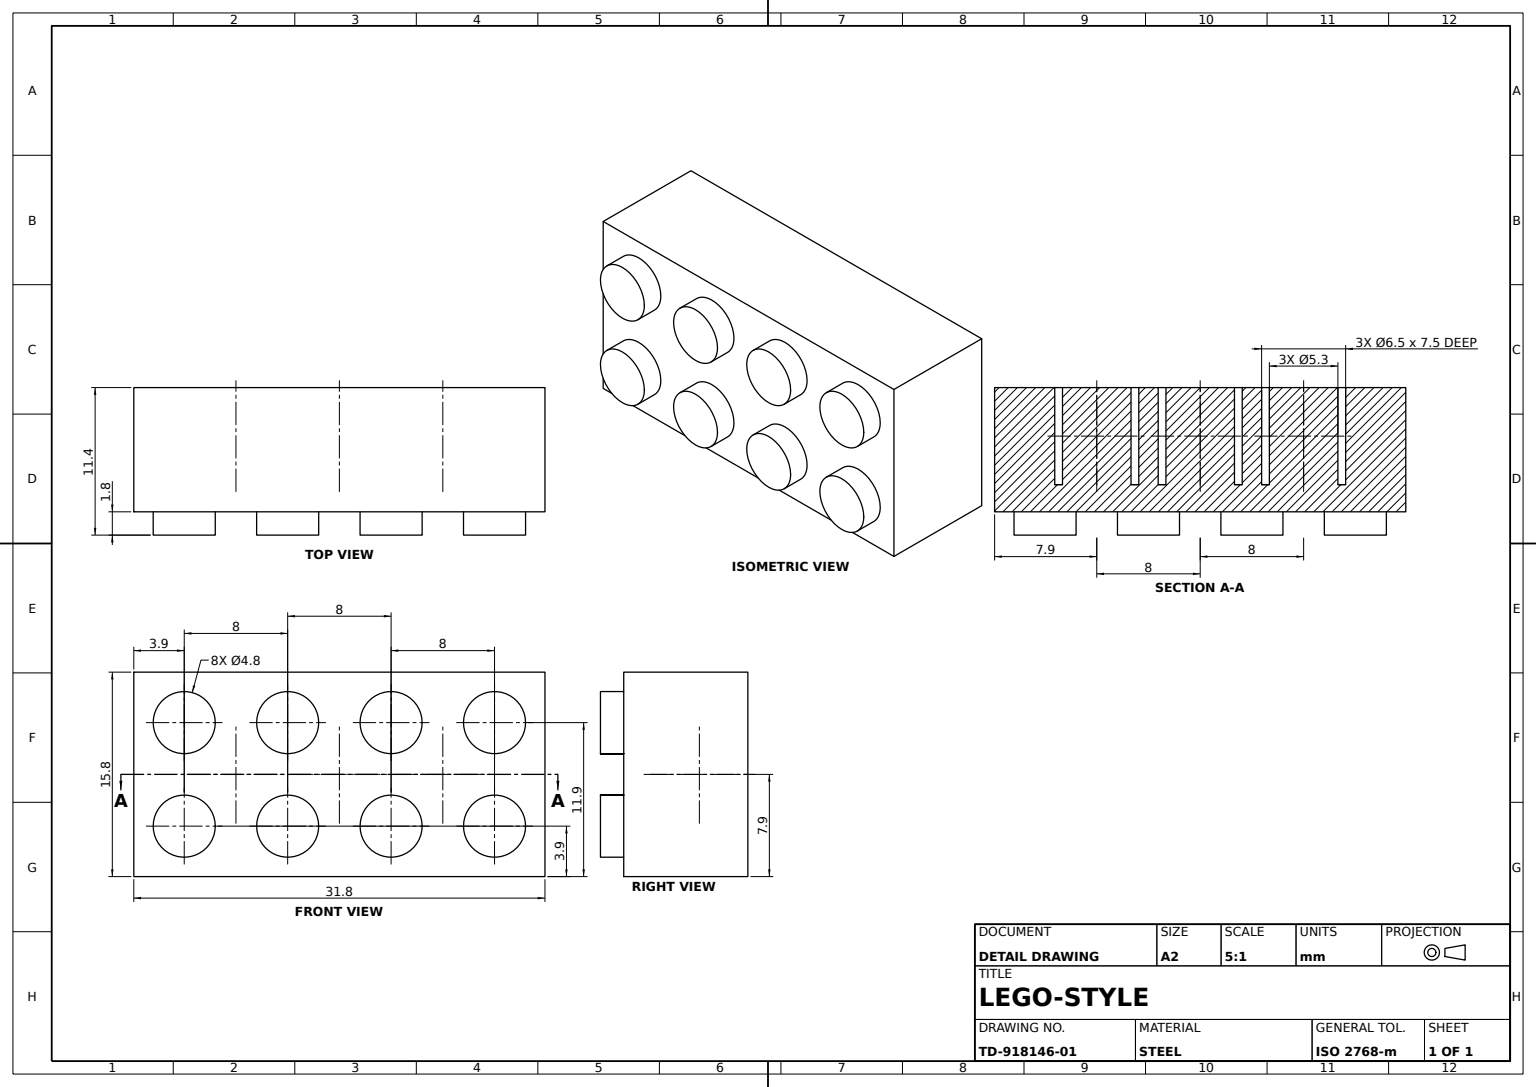
ISO-10303-21;
HEADER;
FILE_DESCRIPTION((''),'2;1');
FILE_NAME('','',(''),(''),'','','');
FILE_SCHEMA(('AUTOMOTIVE_DESIGN'));
ENDSEC;
DATA;
#1=APPLICATION_CONTEXT('');
#2=PRODUCT_CONTEXT('',#1,'mechanical');
#3=PRODUCT('','','',(#2));
#4=PRODUCT_DEFINITION_FORMATION('','',#3);
#5=PRODUCT_DEFINITION_CONTEXT('',#1,'design');
#6=PRODUCT_DEFINITION('','',#4,#5);
#7=PRODUCT_DEFINITION_SHAPE('','',#6);
#8=(LENGTH_UNIT()NAMED_UNIT(*)SI_UNIT(.MILLI.,.METRE.));
#9=(NAMED_UNIT(*)PLANE_ANGLE_UNIT()SI_UNIT($,.RADIAN.));
#10=(NAMED_UNIT(*)SI_UNIT($,.STERADIAN.)SOLID_ANGLE_UNIT());
#11=UNCERTAINTY_MEASURE_WITH_UNIT(LENGTH_MEASURE(1.E-05),#8,'distance_accuracy_value','');
#12=(GEOMETRIC_REPRESENTATION_CONTEXT(3)GLOBAL_UNCERTAINTY_ASSIGNED_CONTEXT((#11))GLOBAL_UNIT_ASSIGNED_CONTEXT((#8,#9,#10))REPRESENTATION_CONTEXT('',''));
#13=CARTESIAN_POINT('',(-4.75,0.,7.5));
#14=VERTEX_POINT('',#13);
#15=CARTESIAN_POINT('',(-11.25,0.,7.5));
#16=VERTEX_POINT('',#15);
#17=CARTESIAN_POINT('',(-8.,0.,7.5));
#18=DIRECTION('',(0.,0.,-1.));
#19=DIRECTION('',(-1.,0.,0.));
#20=AXIS2_PLACEMENT_3D('',#17,#18,#19);
#21=CIRCLE('',#20,3.25);
#22=EDGE_CURVE('',#14,#16,#21,.T.);
#23=ORIENTED_EDGE('',*,*,#22,.T.);
#24=EDGE_CURVE('',#16,#14,#21,.T.);
#25=ORIENTED_EDGE('',*,*,#24,.T.);
#26=EDGE_LOOP('',(#23,#25));
#27=FACE_OUTER_BOUND('',#26,.T.);
#28=CARTESIAN_POINT('',(-5.35,0.,7.5));
#29=VERTEX_POINT('',#28);
#30=CARTESIAN_POINT('',(-10.65,0.,7.5));
#31=VERTEX_POINT('',#30);
#32=CIRCLE('',#20,2.65);
#33=EDGE_CURVE('',#29,#31,#32,.T.);
#34=ORIENTED_EDGE('',*,*,#33,.F.);
#35=EDGE_CURVE('',#31,#29,#32,.T.);
#36=ORIENTED_EDGE('',*,*,#35,.F.);
#37=EDGE_LOOP('',(#34,#36));
#38=FACE_BOUND('',#37,.T.);
#39=PLANE('',#20);
#40=ADVANCED_FACE('',(#27,#38),#39,.T.);
#41=CARTESIAN_POINT('',(-6.4,4.,11.4));
#42=VERTEX_POINT('',#41);
#43=CARTESIAN_POINT('',(-1.6,4.,11.4));
#44=VERTEX_POINT('',#43);
#45=CARTESIAN_POINT('',(-4.,4.,11.4));
#46=DIRECTION('',(0.,0.,1.));
#47=DIRECTION('',(1.,0.,0.));
#48=AXIS2_PLACEMENT_3D('',#45,#46,#47);
#49=CIRCLE('',#48,2.4);
#50=EDGE_CURVE('',#42,#44,#49,.T.);
#51=ORIENTED_EDGE('',*,*,#50,.T.);
#52=EDGE_CURVE('',#44,#42,#49,.T.);
#53=ORIENTED_EDGE('',*,*,#52,.T.);
#54=EDGE_LOOP('',(#51,#53));
#55=FACE_OUTER_BOUND('',#54,.T.);
#56=PLANE('',#48);
#57=ADVANCED_FACE('',(#55),#56,.T.);
#58=CARTESIAN_POINT('',(3.25,0.,0.));
#59=VERTEX_POINT('',#58);
#60=CARTESIAN_POINT('',(3.25,0.,7.5));
#61=VERTEX_POINT('',#60);
#62=CARTESIAN_POINT('',(3.25,0.,-0.000012));
#63=VECTOR('',#46,1000.);
#64=LINE('',#62,#63);
#65=EDGE_CURVE('',#59,#61,#64,.T.);
#66=ORIENTED_EDGE('',*,*,#65,.T.);
#67=CARTESIAN_POINT('',(-3.25,0.,7.5));
#68=VERTEX_POINT('',#67);
#69=CARTESIAN_POINT('',(0.,0.,7.5));
#70=AXIS2_PLACEMENT_3D('',#69,#18,#19);
#71=CIRCLE('',#70,3.25);
#72=EDGE_CURVE('',#68,#61,#71,.T.);
#73=ORIENTED_EDGE('',*,*,#72,.F.);
#74=CARTESIAN_POINT('',(-3.25,0.,0.));
#75=VERTEX_POINT('',#74);
#76=CARTESIAN_POINT('',(-3.25,0.,-0.000012));
#77=LINE('',#76,#63);
#78=EDGE_CURVE('',#75,#68,#77,.T.);
#79=ORIENTED_EDGE('',*,*,#78,.F.);
#80=CARTESIAN_POINT('',(0.,0.,0.));
#81=AXIS2_PLACEMENT_3D('',#80,#18,#47);
#82=CIRCLE('',#81,3.25);
#83=EDGE_CURVE('',#75,#59,#82,.T.);
#84=ORIENTED_EDGE('',*,*,#83,.T.);
#85=EDGE_LOOP('',(#66,#73,#79,#84));
#86=FACE_OUTER_BOUND('',#85,.T.);
#87=CARTESIAN_POINT('',(0.,0.,-0.000012));
#88=AXIS2_PLACEMENT_3D('',#87,#46,#47);
#89=CYLINDRICAL_SURFACE('',#88,3.25);
#90=ADVANCED_FACE('',(#86),#89,.F.);
#91=CARTESIAN_POINT('',(-9.6,-4.,11.4));
#92=VERTEX_POINT('',#91);
#93=CARTESIAN_POINT('',(-14.4,-4.,11.4));
#94=VERTEX_POINT('',#93);
#95=CARTESIAN_POINT('',(-12.,-4.,11.4));
#96=AXIS2_PLACEMENT_3D('',#95,#46,#19);
#97=CIRCLE('',#96,2.4);
#98=EDGE_CURVE('',#92,#94,#97,.T.);
#99=ORIENTED_EDGE('',*,*,#98,.T.);
#100=EDGE_CURVE('',#94,#92,#97,.T.);
#101=ORIENTED_EDGE('',*,*,#100,.T.);
#102=EDGE_LOOP('',(#99,#101));
#103=FACE_OUTER_BOUND('',#102,.T.);
#104=AXIS2_PLACEMENT_3D('',#95,#18,#19);
#105=PLANE('',#104);
#106=ADVANCED_FACE('',(#103),#105,.F.);
#107=CARTESIAN_POINT('',(15.9,7.9,9.6));
#108=VERTEX_POINT('',#107);
#109=CARTESIAN_POINT('',(15.9,7.9,0.));
#110=VERTEX_POINT('',#109);
#111=VECTOR('',#18,1000.);
#112=LINE('',#107,#111);
#113=EDGE_CURVE('',#108,#110,#112,.T.);
#114=ORIENTED_EDGE('',*,*,#113,.T.);
#115=CARTESIAN_POINT('',(-15.9,7.9,0.));
#116=VERTEX_POINT('',#115);
#117=VECTOR('',#47,1000.);
#118=LINE('',#115,#117);
#119=EDGE_CURVE('',#116,#110,#118,.T.);
#120=ORIENTED_EDGE('',*,*,#119,.F.);
#121=CARTESIAN_POINT('',(-15.9,7.9,9.6));
#122=VERTEX_POINT('',#121);
#123=LINE('',#121,#111);
#124=EDGE_CURVE('',#122,#116,#123,.T.);
#125=ORIENTED_EDGE('',*,*,#124,.F.);
#126=LINE('',#121,#117);
#127=EDGE_CURVE('',#122,#108,#126,.T.);
#128=ORIENTED_EDGE('',*,*,#127,.T.);
#129=EDGE_LOOP('',(#114,#120,#125,#128));
#130=FACE_OUTER_BOUND('',#129,.T.);
#131=DIRECTION('',(0.,1.,0.));
#132=AXIS2_PLACEMENT_3D('',#121,#131,#46);
#133=PLANE('',#132);
#134=ADVANCED_FACE('',(#130),#133,.T.);
#135=CARTESIAN_POINT('',(-5.35,0.,0.));
#136=VERTEX_POINT('',#135);
#137=CARTESIAN_POINT('',(-10.65,0.,0.));
#138=VERTEX_POINT('',#137);
#139=CARTESIAN_POINT('',(-8.,0.,0.));
#140=AXIS2_PLACEMENT_3D('',#139,#18,#47);
#141=CIRCLE('',#140,2.65);
#142=EDGE_CURVE('',#136,#138,#141,.T.);
#143=ORIENTED_EDGE('',*,*,#142,.T.);
#144=EDGE_CURVE('',#138,#136,#141,.T.);
#145=ORIENTED_EDGE('',*,*,#144,.T.);
#146=EDGE_LOOP('',(#143,#145));
#147=FACE_OUTER_BOUND('',#146,.T.);
#148=AXIS2_PLACEMENT_3D('',#80,#46,#47);
#149=PLANE('',#148);
#150=ADVANCED_FACE('',(#147),#149,.F.);
#151=CARTESIAN_POINT('',(11.25,0.,0.));
#152=VERTEX_POINT('',#151);
#153=CARTESIAN_POINT('',(4.75,0.,0.));
#154=VERTEX_POINT('',#153);
#155=CARTESIAN_POINT('',(8.,0.,0.));
#156=AXIS2_PLACEMENT_3D('',#155,#18,#47);
#157=CIRCLE('',#156,3.25);
#158=EDGE_CURVE('',#152,#154,#157,.T.);
#159=ORIENTED_EDGE('',*,*,#158,.T.);
#160=CARTESIAN_POINT('',(4.75,0.,7.5));
#161=VERTEX_POINT('',#160);
#162=CARTESIAN_POINT('',(4.75,0.,-0.000012));
#163=LINE('',#162,#63);
#164=EDGE_CURVE('',#154,#161,#163,.T.);
#165=ORIENTED_EDGE('',*,*,#164,.T.);
#166=CARTESIAN_POINT('',(11.25,0.,7.5));
#167=VERTEX_POINT('',#166);
#168=CARTESIAN_POINT('',(8.,0.,7.5));
#169=AXIS2_PLACEMENT_3D('',#168,#18,#19);
#170=CIRCLE('',#169,3.25);
#171=EDGE_CURVE('',#167,#161,#170,.T.);
#172=ORIENTED_EDGE('',*,*,#171,.F.);
#173=CARTESIAN_POINT('',(11.25,0.,-0.000012));
#174=LINE('',#173,#63);
#175=EDGE_CURVE('',#152,#167,#174,.T.);
#176=ORIENTED_EDGE('',*,*,#175,.F.);
#177=EDGE_LOOP('',(#159,#165,#172,#176));
#178=FACE_OUTER_BOUND('',#177,.T.);
#179=CARTESIAN_POINT('',(8.,0.,-0.000012));
#180=AXIS2_PLACEMENT_3D('',#179,#46,#47);
#181=CYLINDRICAL_SURFACE('',#180,3.25);
#182=ADVANCED_FACE('',(#178),#181,.F.);
#183=CARTESIAN_POINT('',(-9.6,4.,11.4));
#184=VERTEX_POINT('',#183);
#185=CARTESIAN_POINT('',(-14.4,4.,11.4));
#186=VERTEX_POINT('',#185);
#187=CARTESIAN_POINT('',(-12.,4.,11.4));
#188=AXIS2_PLACEMENT_3D('',#187,#46,#47);
#189=CIRCLE('',#188,2.4);
#190=EDGE_CURVE('',#184,#186,#189,.T.);
#191=ORIENTED_EDGE('',*,*,#190,.F.);
#192=CARTESIAN_POINT('',(-9.6,4.,9.6));
#193=VERTEX_POINT('',#192);
#194=LINE('',#183,#111);
#195=EDGE_CURVE('',#184,#193,#194,.T.);
#196=ORIENTED_EDGE('',*,*,#195,.T.);
#197=CARTESIAN_POINT('',(-14.4,4.,9.6));
#198=VERTEX_POINT('',#197);
#199=CARTESIAN_POINT('',(-12.,4.,9.6));
#200=AXIS2_PLACEMENT_3D('',#199,#46,#47);
#201=CIRCLE('',#200,2.4);
#202=EDGE_CURVE('',#193,#198,#201,.T.);
#203=ORIENTED_EDGE('',*,*,#202,.T.);
#204=LINE('',#185,#111);
#205=EDGE_CURVE('',#186,#198,#204,.T.);
#206=ORIENTED_EDGE('',*,*,#205,.F.);
#207=EDGE_LOOP('',(#191,#196,#203,#206));
#208=FACE_OUTER_BOUND('',#207,.T.);
#209=AXIS2_PLACEMENT_3D('',#187,#18,#19);
#210=CYLINDRICAL_SURFACE('',#209,2.4);
#211=ADVANCED_FACE('',(#208),#210,.T.);
#212=CARTESIAN_POINT('',(5.35,0.,7.5));
#213=VERTEX_POINT('',#212);
#214=CARTESIAN_POINT('',(10.65,0.,7.5));
#215=VERTEX_POINT('',#214);
#216=CIRCLE('',#169,2.65);
#217=EDGE_CURVE('',#213,#215,#216,.T.);
#218=ORIENTED_EDGE('',*,*,#217,.F.);
#219=EDGE_CURVE('',#215,#213,#216,.T.);
#220=ORIENTED_EDGE('',*,*,#219,.F.);
#221=EDGE_LOOP('',(#218,#220));
#222=FACE_BOUND('',#221,.T.);
#223=ORIENTED_EDGE('',*,*,#171,.T.);
#224=EDGE_CURVE('',#161,#167,#170,.T.);
#225=ORIENTED_EDGE('',*,*,#224,.T.);
#226=EDGE_LOOP('',(#223,#225));
#227=FACE_OUTER_BOUND('',#226,.T.);
#228=PLANE('',#169);
#229=ADVANCED_FACE('',(#222,#227),#228,.T.);
#230=CARTESIAN_POINT('',(-6.4,-4.,11.4));
#231=VERTEX_POINT('',#230);
#232=CARTESIAN_POINT('',(-1.6,-4.,11.4));
#233=VERTEX_POINT('',#232);
#234=CARTESIAN_POINT('',(-4.,-4.,11.4));
#235=AXIS2_PLACEMENT_3D('',#234,#46,#19);
#236=CIRCLE('',#235,2.4);
#237=EDGE_CURVE('',#231,#233,#236,.T.);
#238=ORIENTED_EDGE('',*,*,#237,.T.);
#239=EDGE_CURVE('',#233,#231,#236,.T.);
#240=ORIENTED_EDGE('',*,*,#239,.T.);
#241=EDGE_LOOP('',(#238,#240));
#242=FACE_OUTER_BOUND('',#241,.T.);
#243=AXIS2_PLACEMENT_3D('',#234,#18,#19);
#244=PLANE('',#243);
#245=ADVANCED_FACE('',(#242),#244,.F.);
#246=EDGE_CURVE('',#186,#184,#189,.T.);
#247=ORIENTED_EDGE('',*,*,#246,.T.);
#248=ORIENTED_EDGE('',*,*,#190,.T.);
#249=EDGE_LOOP('',(#247,#248));
#250=FACE_OUTER_BOUND('',#249,.T.);
#251=PLANE('',#188);
#252=ADVANCED_FACE('',(#250),#251,.T.);
#253=CARTESIAN_POINT('',(6.4,-4.,11.4));
#254=VERTEX_POINT('',#253);
#255=CARTESIAN_POINT('',(1.6,-4.,11.4));
#256=VERTEX_POINT('',#255);
#257=CARTESIAN_POINT('',(4.,-4.,11.4));
#258=AXIS2_PLACEMENT_3D('',#257,#46,#19);
#259=CIRCLE('',#258,2.4);
#260=EDGE_CURVE('',#254,#256,#259,.T.);
#261=ORIENTED_EDGE('',*,*,#260,.F.);
#262=CARTESIAN_POINT('',(6.4,-4.,9.6));
#263=VERTEX_POINT('',#262);
#264=LINE('',#253,#111);
#265=EDGE_CURVE('',#254,#263,#264,.T.);
#266=ORIENTED_EDGE('',*,*,#265,.T.);
#267=CARTESIAN_POINT('',(1.6,-4.,9.6));
#268=VERTEX_POINT('',#267);
#269=CARTESIAN_POINT('',(4.,-4.,9.6));
#270=AXIS2_PLACEMENT_3D('',#269,#46,#19);
#271=CIRCLE('',#270,2.4);
#272=EDGE_CURVE('',#263,#268,#271,.T.);
#273=ORIENTED_EDGE('',*,*,#272,.T.);
#274=LINE('',#255,#111);
#275=EDGE_CURVE('',#256,#268,#274,.T.);
#276=ORIENTED_EDGE('',*,*,#275,.F.);
#277=EDGE_LOOP('',(#261,#266,#273,#276));
#278=FACE_OUTER_BOUND('',#277,.T.);
#279=AXIS2_PLACEMENT_3D('',#257,#18,#19);
#280=CYLINDRICAL_SURFACE('',#279,2.4);
#281=ADVANCED_FACE('',(#278),#280,.T.);
#282=CARTESIAN_POINT('',(6.4,4.,11.4));
#283=VERTEX_POINT('',#282);
#284=CARTESIAN_POINT('',(6.4,4.,9.6));
#285=VERTEX_POINT('',#284);
#286=LINE('',#282,#111);
#287=EDGE_CURVE('',#283,#285,#286,.T.);
#288=ORIENTED_EDGE('',*,*,#287,.T.);
#289=CARTESIAN_POINT('',(1.6,4.,9.6));
#290=VERTEX_POINT('',#289);
#291=CARTESIAN_POINT('',(4.,4.,9.6));
#292=AXIS2_PLACEMENT_3D('',#291,#46,#47);
#293=CIRCLE('',#292,2.4);
#294=EDGE_CURVE('',#285,#290,#293,.T.);
#295=ORIENTED_EDGE('',*,*,#294,.T.);
#296=CARTESIAN_POINT('',(1.6,4.,11.4));
#297=VERTEX_POINT('',#296);
#298=LINE('',#296,#111);
#299=EDGE_CURVE('',#297,#290,#298,.T.);
#300=ORIENTED_EDGE('',*,*,#299,.F.);
#301=CARTESIAN_POINT('',(4.,4.,11.4));
#302=AXIS2_PLACEMENT_3D('',#301,#46,#47);
#303=CIRCLE('',#302,2.4);
#304=EDGE_CURVE('',#283,#297,#303,.T.);
#305=ORIENTED_EDGE('',*,*,#304,.F.);
#306=EDGE_LOOP('',(#288,#295,#300,#305));
#307=FACE_OUTER_BOUND('',#306,.T.);
#308=AXIS2_PLACEMENT_3D('',#301,#18,#19);
#309=CYLINDRICAL_SURFACE('',#308,2.4);
#310=ADVANCED_FACE('',(#307),#309,.T.);
#311=ORIENTED_EDGE('',*,*,#275,.T.);
#312=EDGE_CURVE('',#268,#263,#271,.T.);
#313=ORIENTED_EDGE('',*,*,#312,.T.);
#314=ORIENTED_EDGE('',*,*,#265,.F.);
#315=EDGE_CURVE('',#256,#254,#259,.T.);
#316=ORIENTED_EDGE('',*,*,#315,.F.);
#317=EDGE_LOOP('',(#311,#313,#314,#316));
#318=FACE_OUTER_BOUND('',#317,.T.);
#319=ADVANCED_FACE('',(#318),#280,.T.);
#320=ORIENTED_EDGE('',*,*,#113,.F.);
#321=CARTESIAN_POINT('',(15.9,-7.9,9.6));
#322=VERTEX_POINT('',#321);
#323=DIRECTION('',(0.,-1.,0.));
#324=VECTOR('',#323,1000.);
#325=LINE('',#107,#324);
#326=EDGE_CURVE('',#108,#322,#325,.T.);
#327=ORIENTED_EDGE('',*,*,#326,.T.);
#328=CARTESIAN_POINT('',(15.9,-7.9,0.));
#329=VERTEX_POINT('',#328);
#330=LINE('',#321,#111);
#331=EDGE_CURVE('',#322,#329,#330,.T.);
#332=ORIENTED_EDGE('',*,*,#331,.T.);
#333=LINE('',#109,#324);
#334=EDGE_CURVE('',#110,#329,#333,.T.);
#335=ORIENTED_EDGE('',*,*,#334,.F.);
#336=EDGE_LOOP('',(#320,#327,#332,#335));
#337=FACE_OUTER_BOUND('',#336,.T.);
#338=AXIS2_PLACEMENT_3D('',#107,#47,#18);
#339=PLANE('',#338);
#340=ADVANCED_FACE('',(#337),#339,.T.);
#341=CARTESIAN_POINT('',(14.4,4.,9.6));
#342=VERTEX_POINT('',#341);
#343=CARTESIAN_POINT('',(9.6,4.,9.6));
#344=VERTEX_POINT('',#343);
#345=CARTESIAN_POINT('',(12.,4.,9.6));
#346=AXIS2_PLACEMENT_3D('',#345,#46,#47);
#347=CIRCLE('',#346,2.4);
#348=EDGE_CURVE('',#342,#344,#347,.T.);
#349=ORIENTED_EDGE('',*,*,#348,.T.);
#350=CARTESIAN_POINT('',(9.6,4.,11.4));
#351=VERTEX_POINT('',#350);
#352=LINE('',#350,#111);
#353=EDGE_CURVE('',#351,#344,#352,.T.);
#354=ORIENTED_EDGE('',*,*,#353,.F.);
#355=CARTESIAN_POINT('',(14.4,4.,11.4));
#356=VERTEX_POINT('',#355);
#357=CARTESIAN_POINT('',(12.,4.,11.4));
#358=AXIS2_PLACEMENT_3D('',#357,#46,#47);
#359=CIRCLE('',#358,2.4);
#360=EDGE_CURVE('',#356,#351,#359,.T.);
#361=ORIENTED_EDGE('',*,*,#360,.F.);
#362=LINE('',#355,#111);
#363=EDGE_CURVE('',#356,#342,#362,.T.);
#364=ORIENTED_EDGE('',*,*,#363,.T.);
#365=EDGE_LOOP('',(#349,#354,#361,#364));
#366=FACE_OUTER_BOUND('',#365,.T.);
#367=AXIS2_PLACEMENT_3D('',#357,#18,#19);
#368=CYLINDRICAL_SURFACE('',#367,2.4);
#369=ADVANCED_FACE('',(#366),#368,.T.);
#370=CARTESIAN_POINT('',(2.65,0.,0.));
#371=VERTEX_POINT('',#370);
#372=CARTESIAN_POINT('',(2.65,0.,7.5));
#373=VERTEX_POINT('',#372);
#374=CARTESIAN_POINT('',(2.65,0.,-0.000012));
#375=LINE('',#374,#63);
#376=EDGE_CURVE('',#371,#373,#375,.T.);
#377=ORIENTED_EDGE('',*,*,#376,.F.);
#378=CARTESIAN_POINT('',(-2.65,0.,0.));
#379=VERTEX_POINT('',#378);
#380=CIRCLE('',#81,2.65);
#381=EDGE_CURVE('',#379,#371,#380,.T.);
#382=ORIENTED_EDGE('',*,*,#381,.F.);
#383=CARTESIAN_POINT('',(-2.65,0.,7.5));
#384=VERTEX_POINT('',#383);
#385=CARTESIAN_POINT('',(-2.65,0.,-0.000012));
#386=LINE('',#385,#63);
#387=EDGE_CURVE('',#379,#384,#386,.T.);
#388=ORIENTED_EDGE('',*,*,#387,.T.);
#389=CIRCLE('',#70,2.65);
#390=EDGE_CURVE('',#384,#373,#389,.T.);
#391=ORIENTED_EDGE('',*,*,#390,.T.);
#392=EDGE_LOOP('',(#377,#382,#388,#391));
#393=FACE_OUTER_BOUND('',#392,.T.);
#394=CYLINDRICAL_SURFACE('',#88,2.65);
#395=ADVANCED_FACE('',(#393),#394,.T.);
#396=CARTESIAN_POINT('',(14.4,-4.,11.4));
#397=VERTEX_POINT('',#396);
#398=CARTESIAN_POINT('',(9.6,-4.,11.4));
#399=VERTEX_POINT('',#398);
#400=CARTESIAN_POINT('',(12.,-4.,11.4));
#401=AXIS2_PLACEMENT_3D('',#400,#46,#19);
#402=CIRCLE('',#401,2.4);
#403=EDGE_CURVE('',#397,#399,#402,.T.);
#404=ORIENTED_EDGE('',*,*,#403,.F.);
#405=CARTESIAN_POINT('',(14.4,-4.,9.6));
#406=VERTEX_POINT('',#405);
#407=LINE('',#396,#111);
#408=EDGE_CURVE('',#397,#406,#407,.T.);
#409=ORIENTED_EDGE('',*,*,#408,.T.);
#410=CARTESIAN_POINT('',(9.6,-4.,9.6));
#411=VERTEX_POINT('',#410);
#412=CARTESIAN_POINT('',(12.,-4.,9.6));
#413=AXIS2_PLACEMENT_3D('',#412,#46,#19);
#414=CIRCLE('',#413,2.4);
#415=EDGE_CURVE('',#406,#411,#414,.T.);
#416=ORIENTED_EDGE('',*,*,#415,.T.);
#417=LINE('',#398,#111);
#418=EDGE_CURVE('',#399,#411,#417,.T.);
#419=ORIENTED_EDGE('',*,*,#418,.F.);
#420=EDGE_LOOP('',(#404,#409,#416,#419));
#421=FACE_OUTER_BOUND('',#420,.T.);
#422=AXIS2_PLACEMENT_3D('',#400,#18,#19);
#423=CYLINDRICAL_SURFACE('',#422,2.4);
#424=ADVANCED_FACE('',(#421),#423,.T.);
#425=ORIENTED_EDGE('',*,*,#299,.T.);
#426=EDGE_CURVE('',#290,#285,#293,.T.);
#427=ORIENTED_EDGE('',*,*,#426,.T.);
#428=ORIENTED_EDGE('',*,*,#287,.F.);
#429=EDGE_CURVE('',#297,#283,#303,.T.);
#430=ORIENTED_EDGE('',*,*,#429,.F.);
#431=EDGE_LOOP('',(#425,#427,#428,#430));
#432=FACE_OUTER_BOUND('',#431,.T.);
#433=ADVANCED_FACE('',(#432),#309,.T.);
#434=ORIENTED_EDGE('',*,*,#304,.T.);
#435=ORIENTED_EDGE('',*,*,#429,.T.);
#436=EDGE_LOOP('',(#434,#435));
#437=FACE_OUTER_BOUND('',#436,.T.);
#438=PLANE('',#302);
#439=ADVANCED_FACE('',(#437),#438,.T.);
#440=ORIENTED_EDGE('',*,*,#217,.T.);
#441=CARTESIAN_POINT('',(10.65,0.,0.));
#442=VERTEX_POINT('',#441);
#443=CARTESIAN_POINT('',(10.65,0.,-0.000012));
#444=LINE('',#443,#63);
#445=EDGE_CURVE('',#442,#215,#444,.T.);
#446=ORIENTED_EDGE('',*,*,#445,.F.);
#447=CARTESIAN_POINT('',(5.35,0.,0.));
#448=VERTEX_POINT('',#447);
#449=CIRCLE('',#156,2.65);
#450=EDGE_CURVE('',#448,#442,#449,.T.);
#451=ORIENTED_EDGE('',*,*,#450,.F.);
#452=CARTESIAN_POINT('',(5.35,0.,-0.000012));
#453=LINE('',#452,#63);
#454=EDGE_CURVE('',#448,#213,#453,.T.);
#455=ORIENTED_EDGE('',*,*,#454,.T.);
#456=EDGE_LOOP('',(#440,#446,#451,#455));
#457=FACE_OUTER_BOUND('',#456,.T.);
#458=CYLINDRICAL_SURFACE('',#180,2.65);
#459=ADVANCED_FACE('',(#457),#458,.T.);
#460=EDGE_CURVE('',#371,#379,#380,.T.);
#461=ORIENTED_EDGE('',*,*,#460,.T.);
#462=ORIENTED_EDGE('',*,*,#381,.T.);
#463=EDGE_LOOP('',(#461,#462));
#464=FACE_OUTER_BOUND('',#463,.T.);
#465=ADVANCED_FACE('',(#464),#149,.F.);
#466=CARTESIAN_POINT('',(-11.25,0.,0.));
#467=VERTEX_POINT('',#466);
#468=CARTESIAN_POINT('',(-11.25,0.,-0.000012));
#469=LINE('',#468,#63);
#470=EDGE_CURVE('',#467,#16,#469,.T.);
#471=ORIENTED_EDGE('',*,*,#470,.F.);
#472=CARTESIAN_POINT('',(-4.75,0.,0.));
#473=VERTEX_POINT('',#472);
#474=CIRCLE('',#140,3.25);
#475=EDGE_CURVE('',#467,#473,#474,.T.);
#476=ORIENTED_EDGE('',*,*,#475,.T.);
#477=CARTESIAN_POINT('',(-4.75,0.,-0.000012));
#478=LINE('',#477,#63);
#479=EDGE_CURVE('',#473,#14,#478,.T.);
#480=ORIENTED_EDGE('',*,*,#479,.T.);
#481=ORIENTED_EDGE('',*,*,#24,.F.);
#482=EDGE_LOOP('',(#471,#476,#480,#481));
#483=FACE_OUTER_BOUND('',#482,.T.);
#484=CARTESIAN_POINT('',(-8.,0.,-0.000012));
#485=AXIS2_PLACEMENT_3D('',#484,#46,#47);
#486=CYLINDRICAL_SURFACE('',#485,3.25);
#487=ADVANCED_FACE('',(#483),#486,.F.);
#488=CARTESIAN_POINT('',(-6.4,-4.,9.6));
#489=VERTEX_POINT('',#488);
#490=LINE('',#230,#111);
#491=EDGE_CURVE('',#231,#489,#490,.T.);
#492=ORIENTED_EDGE('',*,*,#491,.T.);
#493=CARTESIAN_POINT('',(-1.6,-4.,9.6));
#494=VERTEX_POINT('',#493);
#495=CARTESIAN_POINT('',(-4.,-4.,9.6));
#496=AXIS2_PLACEMENT_3D('',#495,#46,#19);
#497=CIRCLE('',#496,2.4);
#498=EDGE_CURVE('',#489,#494,#497,.T.);
#499=ORIENTED_EDGE('',*,*,#498,.T.);
#500=LINE('',#232,#111);
#501=EDGE_CURVE('',#233,#494,#500,.T.);
#502=ORIENTED_EDGE('',*,*,#501,.F.);
#503=ORIENTED_EDGE('',*,*,#237,.F.);
#504=EDGE_LOOP('',(#492,#499,#502,#503));
#505=FACE_OUTER_BOUND('',#504,.T.);
#506=CYLINDRICAL_SURFACE('',#243,2.4);
#507=ADVANCED_FACE('',(#505),#506,.T.);
#508=CARTESIAN_POINT('',(-15.9,-7.9,9.6));
#509=VERTEX_POINT('',#508);
#510=LINE('',#121,#324);
#511=EDGE_CURVE('',#122,#509,#510,.T.);
#512=ORIENTED_EDGE('',*,*,#511,.F.);
#513=ORIENTED_EDGE('',*,*,#124,.T.);
#514=CARTESIAN_POINT('',(-15.9,-7.9,0.));
#515=VERTEX_POINT('',#514);
#516=LINE('',#115,#324);
#517=EDGE_CURVE('',#116,#515,#516,.T.);
#518=ORIENTED_EDGE('',*,*,#517,.T.);
#519=LINE('',#508,#111);
#520=EDGE_CURVE('',#509,#515,#519,.T.);
#521=ORIENTED_EDGE('',*,*,#520,.F.);
#522=EDGE_LOOP('',(#512,#513,#518,#521));
#523=FACE_OUTER_BOUND('',#522,.T.);
#524=AXIS2_PLACEMENT_3D('',#121,#47,#131);
#525=PLANE('',#524);
#526=ADVANCED_FACE('',(#523),#525,.F.);
#527=EDGE_CURVE('',#351,#356,#359,.T.);
#528=ORIENTED_EDGE('',*,*,#527,.T.);
#529=ORIENTED_EDGE('',*,*,#360,.T.);
#530=EDGE_LOOP('',(#528,#529));
#531=FACE_OUTER_BOUND('',#530,.T.);
#532=PLANE('',#358);
#533=ADVANCED_FACE('',(#531),#532,.T.);
#534=CARTESIAN_POINT('',(-14.4,-4.,9.6));
#535=VERTEX_POINT('',#534);
#536=CARTESIAN_POINT('',(-9.6,-4.,9.6));
#537=VERTEX_POINT('',#536);
#538=CARTESIAN_POINT('',(-12.,-4.,9.6));
#539=AXIS2_PLACEMENT_3D('',#538,#46,#19);
#540=CIRCLE('',#539,2.4);
#541=EDGE_CURVE('',#535,#537,#540,.T.);
#542=ORIENTED_EDGE('',*,*,#541,.F.);
#543=EDGE_CURVE('',#537,#535,#540,.T.);
#544=ORIENTED_EDGE('',*,*,#543,.F.);
#545=EDGE_LOOP('',(#542,#544));
#546=FACE_BOUND('',#545,.T.);
#547=ORIENTED_EDGE('',*,*,#272,.F.);
#548=ORIENTED_EDGE('',*,*,#312,.F.);
#549=EDGE_LOOP('',(#547,#548));
#550=FACE_BOUND('',#549,.T.);
#551=EDGE_CURVE('',#344,#342,#347,.T.);
#552=ORIENTED_EDGE('',*,*,#551,.F.);
#553=ORIENTED_EDGE('',*,*,#348,.F.);
#554=EDGE_LOOP('',(#552,#553));
#555=FACE_BOUND('',#554,.T.);
#556=CARTESIAN_POINT('',(-1.6,4.,9.6));
#557=VERTEX_POINT('',#556);
#558=CARTESIAN_POINT('',(-6.4,4.,9.6));
#559=VERTEX_POINT('',#558);
#560=CARTESIAN_POINT('',(-4.,4.,9.6));
#561=AXIS2_PLACEMENT_3D('',#560,#46,#47);
#562=CIRCLE('',#561,2.4);
#563=EDGE_CURVE('',#557,#559,#562,.T.);
#564=ORIENTED_EDGE('',*,*,#563,.F.);
#565=EDGE_CURVE('',#559,#557,#562,.T.);
#566=ORIENTED_EDGE('',*,*,#565,.F.);
#567=EDGE_LOOP('',(#564,#566));
#568=FACE_BOUND('',#567,.T.);
#569=ORIENTED_EDGE('',*,*,#326,.F.);
#570=ORIENTED_EDGE('',*,*,#127,.F.);
#571=ORIENTED_EDGE('',*,*,#511,.T.);
#572=LINE('',#508,#117);
#573=EDGE_CURVE('',#509,#322,#572,.T.);
#574=ORIENTED_EDGE('',*,*,#573,.T.);
#575=EDGE_LOOP('',(#569,#570,#571,#574));
#576=FACE_OUTER_BOUND('',#575,.T.);
#577=EDGE_CURVE('',#198,#193,#201,.T.);
#578=ORIENTED_EDGE('',*,*,#577,.F.);
#579=ORIENTED_EDGE('',*,*,#202,.F.);
#580=EDGE_LOOP('',(#578,#579));
#581=FACE_BOUND('',#580,.T.);
#582=ORIENTED_EDGE('',*,*,#415,.F.);
#583=EDGE_CURVE('',#411,#406,#414,.T.);
#584=ORIENTED_EDGE('',*,*,#583,.F.);
#585=EDGE_LOOP('',(#582,#584));
#586=FACE_BOUND('',#585,.T.);
#587=EDGE_CURVE('',#494,#489,#497,.T.);
#588=ORIENTED_EDGE('',*,*,#587,.F.);
#589=ORIENTED_EDGE('',*,*,#498,.F.);
#590=EDGE_LOOP('',(#588,#589));
#591=FACE_BOUND('',#590,.T.);
#592=ORIENTED_EDGE('',*,*,#294,.F.);
#593=ORIENTED_EDGE('',*,*,#426,.F.);
#594=EDGE_LOOP('',(#592,#593));
#595=FACE_BOUND('',#594,.T.);
#596=CARTESIAN_POINT('',(0.,0.,9.6));
#597=AXIS2_PLACEMENT_3D('',#596,#46,#47);
#598=PLANE('',#597);
#599=ADVANCED_FACE('',(#546,#550,#555,#568,#576,#581,#586,#591,#595),#598,.T.);
#600=EDGE_CURVE('',#373,#384,#389,.T.);
#601=ORIENTED_EDGE('',*,*,#600,.F.);
#602=ORIENTED_EDGE('',*,*,#390,.F.);
#603=EDGE_LOOP('',(#601,#602));
#604=FACE_BOUND('',#603,.T.);
#605=ORIENTED_EDGE('',*,*,#72,.T.);
#606=EDGE_CURVE('',#61,#68,#71,.T.);
#607=ORIENTED_EDGE('',*,*,#606,.T.);
#608=EDGE_LOOP('',(#605,#607));
#609=FACE_OUTER_BOUND('',#608,.T.);
#610=PLANE('',#70);
#611=ADVANCED_FACE('',(#604,#609),#610,.T.);
#612=EDGE_CURVE('',#399,#397,#402,.T.);
#613=ORIENTED_EDGE('',*,*,#612,.F.);
#614=ORIENTED_EDGE('',*,*,#418,.T.);
#615=ORIENTED_EDGE('',*,*,#583,.T.);
#616=ORIENTED_EDGE('',*,*,#408,.F.);
#617=EDGE_LOOP('',(#613,#614,#615,#616));
#618=FACE_OUTER_BOUND('',#617,.T.);
#619=ADVANCED_FACE('',(#618),#423,.T.);
#620=ORIENTED_EDGE('',*,*,#450,.T.);
#621=EDGE_CURVE('',#442,#448,#449,.T.);
#622=ORIENTED_EDGE('',*,*,#621,.T.);
#623=EDGE_LOOP('',(#620,#622));
#624=FACE_OUTER_BOUND('',#623,.T.);
#625=ADVANCED_FACE('',(#624),#149,.F.);
#626=ORIENTED_EDGE('',*,*,#363,.F.);
#627=ORIENTED_EDGE('',*,*,#527,.F.);
#628=ORIENTED_EDGE('',*,*,#353,.T.);
#629=ORIENTED_EDGE('',*,*,#551,.T.);
#630=EDGE_LOOP('',(#626,#627,#628,#629));
#631=FACE_OUTER_BOUND('',#630,.T.);
#632=ADVANCED_FACE('',(#631),#368,.T.);
#633=CARTESIAN_POINT('',(-10.65,0.,-0.000012));
#634=LINE('',#633,#63);
#635=EDGE_CURVE('',#138,#31,#634,.T.);
#636=ORIENTED_EDGE('',*,*,#635,.T.);
#637=ORIENTED_EDGE('',*,*,#35,.T.);
#638=CARTESIAN_POINT('',(-5.35,0.,-0.000012));
#639=LINE('',#638,#63);
#640=EDGE_CURVE('',#136,#29,#639,.T.);
#641=ORIENTED_EDGE('',*,*,#640,.F.);
#642=ORIENTED_EDGE('',*,*,#144,.F.);
#643=EDGE_LOOP('',(#636,#637,#641,#642));
#644=FACE_OUTER_BOUND('',#643,.T.);
#645=CYLINDRICAL_SURFACE('',#485,2.65);
#646=ADVANCED_FACE('',(#644),#645,.T.);
#647=ORIENTED_EDGE('',*,*,#260,.T.);
#648=ORIENTED_EDGE('',*,*,#315,.T.);
#649=EDGE_LOOP('',(#647,#648));
#650=FACE_OUTER_BOUND('',#649,.T.);
#651=PLANE('',#279);
#652=ADVANCED_FACE('',(#650),#651,.F.);
#653=LINE('',#93,#111);
#654=EDGE_CURVE('',#94,#535,#653,.T.);
#655=ORIENTED_EDGE('',*,*,#654,.T.);
#656=ORIENTED_EDGE('',*,*,#541,.T.);
#657=LINE('',#91,#111);
#658=EDGE_CURVE('',#92,#537,#657,.T.);
#659=ORIENTED_EDGE('',*,*,#658,.F.);
#660=ORIENTED_EDGE('',*,*,#100,.F.);
#661=EDGE_LOOP('',(#655,#656,#659,#660));
#662=FACE_OUTER_BOUND('',#661,.T.);
#663=CYLINDRICAL_SURFACE('',#104,2.4);
#664=ADVANCED_FACE('',(#662),#663,.T.);
#665=ORIENTED_EDGE('',*,*,#606,.F.);
#666=ORIENTED_EDGE('',*,*,#65,.F.);
#667=EDGE_CURVE('',#59,#75,#82,.T.);
#668=ORIENTED_EDGE('',*,*,#667,.T.);
#669=ORIENTED_EDGE('',*,*,#78,.T.);
#670=EDGE_LOOP('',(#665,#666,#668,#669));
#671=FACE_OUTER_BOUND('',#670,.T.);
#672=ADVANCED_FACE('',(#671),#89,.F.);
#673=ORIENTED_EDGE('',*,*,#658,.T.);
#674=ORIENTED_EDGE('',*,*,#543,.T.);
#675=ORIENTED_EDGE('',*,*,#654,.F.);
#676=ORIENTED_EDGE('',*,*,#98,.F.);
#677=EDGE_LOOP('',(#673,#674,#675,#676));
#678=FACE_OUTER_BOUND('',#677,.T.);
#679=ADVANCED_FACE('',(#678),#663,.T.);
#680=ORIENTED_EDGE('',*,*,#387,.F.);
#681=ORIENTED_EDGE('',*,*,#460,.F.);
#682=ORIENTED_EDGE('',*,*,#376,.T.);
#683=ORIENTED_EDGE('',*,*,#600,.T.);
#684=EDGE_LOOP('',(#680,#681,#682,#683));
#685=FACE_OUTER_BOUND('',#684,.T.);
#686=ADVANCED_FACE('',(#685),#394,.T.);
#687=ORIENTED_EDGE('',*,*,#219,.T.);
#688=ORIENTED_EDGE('',*,*,#454,.F.);
#689=ORIENTED_EDGE('',*,*,#621,.F.);
#690=ORIENTED_EDGE('',*,*,#445,.T.);
#691=EDGE_LOOP('',(#687,#688,#689,#690));
#692=FACE_OUTER_BOUND('',#691,.T.);
#693=ADVANCED_FACE('',(#692),#458,.T.);
#694=ORIENTED_EDGE('',*,*,#195,.F.);
#695=ORIENTED_EDGE('',*,*,#246,.F.);
#696=ORIENTED_EDGE('',*,*,#205,.T.);
#697=ORIENTED_EDGE('',*,*,#577,.T.);
#698=EDGE_LOOP('',(#694,#695,#696,#697));
#699=FACE_OUTER_BOUND('',#698,.T.);
#700=ADVANCED_FACE('',(#699),#210,.T.);
#701=ORIENTED_EDGE('',*,*,#164,.F.);
#702=EDGE_CURVE('',#154,#152,#157,.T.);
#703=ORIENTED_EDGE('',*,*,#702,.T.);
#704=ORIENTED_EDGE('',*,*,#175,.T.);
#705=ORIENTED_EDGE('',*,*,#224,.F.);
#706=EDGE_LOOP('',(#701,#703,#704,#705));
#707=FACE_OUTER_BOUND('',#706,.T.);
#708=ADVANCED_FACE('',(#707),#181,.F.);
#709=ORIENTED_EDGE('',*,*,#52,.F.);
#710=LINE('',#43,#111);
#711=EDGE_CURVE('',#44,#557,#710,.T.);
#712=ORIENTED_EDGE('',*,*,#711,.T.);
#713=ORIENTED_EDGE('',*,*,#563,.T.);
#714=LINE('',#41,#111);
#715=EDGE_CURVE('',#42,#559,#714,.T.);
#716=ORIENTED_EDGE('',*,*,#715,.F.);
#717=EDGE_LOOP('',(#709,#712,#713,#716));
#718=FACE_OUTER_BOUND('',#717,.T.);
#719=AXIS2_PLACEMENT_3D('',#45,#18,#19);
#720=CYLINDRICAL_SURFACE('',#719,2.4);
#721=ADVANCED_FACE('',(#718),#720,.T.);
#722=ORIENTED_EDGE('',*,*,#491,.F.);
#723=ORIENTED_EDGE('',*,*,#239,.F.);
#724=ORIENTED_EDGE('',*,*,#501,.T.);
#725=ORIENTED_EDGE('',*,*,#587,.T.);
#726=EDGE_LOOP('',(#722,#723,#724,#725));
#727=FACE_OUTER_BOUND('',#726,.T.);
#728=ADVANCED_FACE('',(#727),#506,.T.);
#729=ORIENTED_EDGE('',*,*,#640,.T.);
#730=ORIENTED_EDGE('',*,*,#33,.T.);
#731=ORIENTED_EDGE('',*,*,#635,.F.);
#732=ORIENTED_EDGE('',*,*,#142,.F.);
#733=EDGE_LOOP('',(#729,#730,#731,#732));
#734=FACE_OUTER_BOUND('',#733,.T.);
#735=ADVANCED_FACE('',(#734),#645,.T.);
#736=ORIENTED_EDGE('',*,*,#573,.F.);
#737=ORIENTED_EDGE('',*,*,#520,.T.);
#738=LINE('',#514,#117);
#739=EDGE_CURVE('',#515,#329,#738,.T.);
#740=ORIENTED_EDGE('',*,*,#739,.T.);
#741=ORIENTED_EDGE('',*,*,#331,.F.);
#742=EDGE_LOOP('',(#736,#737,#740,#741));
#743=FACE_OUTER_BOUND('',#742,.T.);
#744=AXIS2_PLACEMENT_3D('',#508,#131,#46);
#745=PLANE('',#744);
#746=ADVANCED_FACE('',(#743),#745,.F.);
#747=ORIENTED_EDGE('',*,*,#565,.T.);
#748=ORIENTED_EDGE('',*,*,#711,.F.);
#749=ORIENTED_EDGE('',*,*,#50,.F.);
#750=ORIENTED_EDGE('',*,*,#715,.T.);
#751=EDGE_LOOP('',(#747,#748,#749,#750));
#752=FACE_OUTER_BOUND('',#751,.T.);
#753=ADVANCED_FACE('',(#752),#720,.T.);
#754=ORIENTED_EDGE('',*,*,#334,.T.);
#755=ORIENTED_EDGE('',*,*,#739,.F.);
#756=ORIENTED_EDGE('',*,*,#517,.F.);
#757=ORIENTED_EDGE('',*,*,#119,.T.);
#758=EDGE_LOOP('',(#754,#755,#756,#757));
#759=FACE_OUTER_BOUND('',#758,.T.);
#760=ORIENTED_EDGE('',*,*,#83,.F.);
#761=ORIENTED_EDGE('',*,*,#667,.F.);
#762=EDGE_LOOP('',(#760,#761));
#763=FACE_BOUND('',#762,.T.);
#764=ORIENTED_EDGE('',*,*,#158,.F.);
#765=ORIENTED_EDGE('',*,*,#702,.F.);
#766=EDGE_LOOP('',(#764,#765));
#767=FACE_BOUND('',#766,.T.);
#768=ORIENTED_EDGE('',*,*,#475,.F.);
#769=EDGE_CURVE('',#473,#467,#474,.T.);
#770=ORIENTED_EDGE('',*,*,#769,.F.);
#771=EDGE_LOOP('',(#768,#770));
#772=FACE_BOUND('',#771,.T.);
#773=ADVANCED_FACE('',(#759,#763,#767,#772),#149,.F.);
#774=ORIENTED_EDGE('',*,*,#403,.T.);
#775=ORIENTED_EDGE('',*,*,#612,.T.);
#776=EDGE_LOOP('',(#774,#775));
#777=FACE_OUTER_BOUND('',#776,.T.);
#778=PLANE('',#422);
#779=ADVANCED_FACE('',(#777),#778,.F.);
#780=ORIENTED_EDGE('',*,*,#479,.F.);
#781=ORIENTED_EDGE('',*,*,#769,.T.);
#782=ORIENTED_EDGE('',*,*,#470,.T.);
#783=ORIENTED_EDGE('',*,*,#22,.F.);
#784=EDGE_LOOP('',(#780,#781,#782,#783));
#785=FACE_OUTER_BOUND('',#784,.T.);
#786=ADVANCED_FACE('',(#785),#486,.F.);
#787=CLOSED_SHELL('',(#40,#57,#90,#106,#134,#150,#182,#211,#229,#245,#252,#281,#310,#319,#340,#369,#395,#424,#433,#439,#459,#465,#487,#507,#526,#533,#599,#611,#619,#625,#632,#646,#652,#664,#672,#679,#686,#693,#700,#708,#721,#728,#735,#746,#753,#773,#779,#786));
#788=MANIFOLD_SOLID_BREP('',#787);
#789=ADVANCED_BREP_SHAPE_REPRESENTATION('',(#788),#12);
#790=SHAPE_DEFINITION_REPRESENTATION(#7,#789);
ENDSEC;
END-ISO-10303-21;
